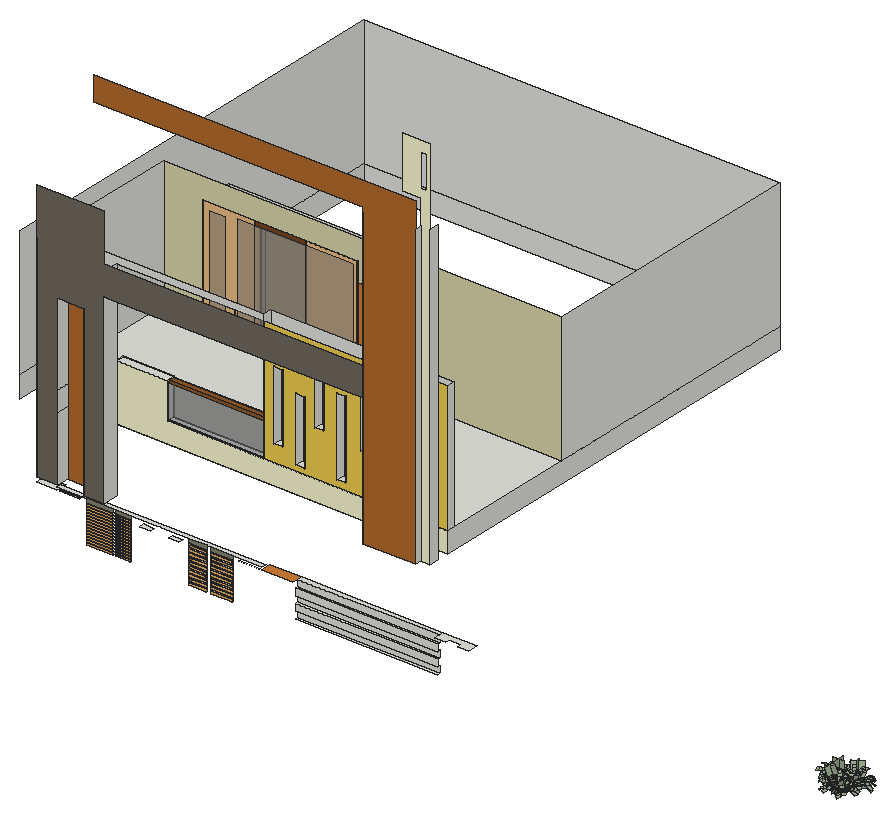
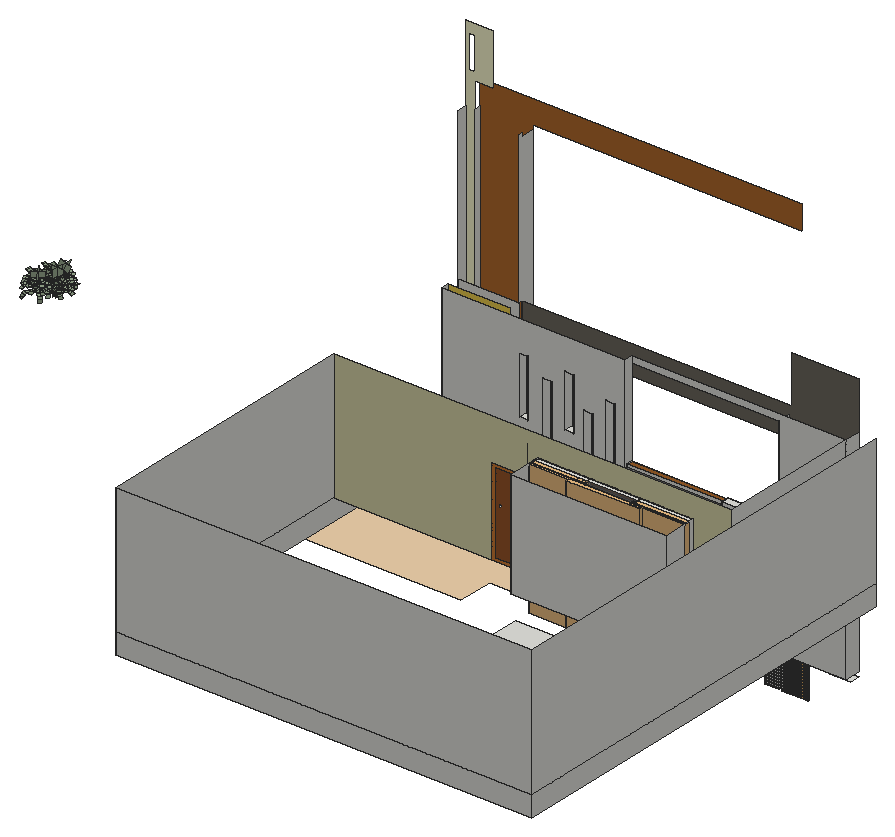
# SketchUp Ruby script. Lengths in inches.
U = 1.inch
M = Sketchup.active_model
def pt(a) = Geom::Point3d.new(a.map { |v| v * U })
def face(e, loops, mat)
  f = e.add_face(loops[0].map { |a| pt(a) })
  loops[1..].each { |l| e.add_face(l.map { |a| pt(a) }).erase! }
  f.material = f.back_material = mat if mat
  f
end
# faces: each face lists its corners as indices into pts; further lists are holes
def faces(e, pts, list, mat = nil) = list.each { |f| face(e, (f[0].is_a?(Array) ? f : [f]).map { |l| l.map { |i| pts[i] } }, mat) }
# xy, xz, yz: faces in a plane at the given z, y or x. An outline is a flat list of corners, or four numbers for a rectangle; further outlines are holes
def ring(l) = l.size == 4 ? [[l[0], l[1]], [l[2], l[1]], [l[2], l[3]], [l[0], l[3]]] : l.each_slice(2).to_a
def flat(e, list, mat, &to3) = list.each { |f| face(e, (f[0].is_a?(Array) ? f : [f]).map { |l| ring(l).map { |u, v| to3.(u, v) } }, mat) }
def xy(e, z, list, mat = nil) = flat(e, list, mat) { |x, y| [x, y, z] }
def xz(e, y, list, mat = nil) = flat(e, list, mat) { |x, z| [x, y, z] }
def yz(e, x, list, mat = nil) = flat(e, list, mat) { |y, z| [x, y, z] }
def lines(e, pts, list) = list.each { |a, b| e.add_line(pt(pts[a]), pt(pts[b])) }
# prism: a flat outline (further loops are holes) pulled along v
def prism(e, loops, v, mat = nil)
  f = face(e, loops, mat); d = Geom::Vector3d.new(v.map { |x| x * U })
  f.pushpull(f.normal.samedirection?(d) ? d.length : -d.length)
end
def box(e, o, s, mat = nil) = prism(e, [[o, [o[0] + s[0], o[1], o[2]], [o[0] + s[0], o[1] + s[1], o[2]], [o[0], o[1] + s[1], o[2]]]], [0, 0, s[2]], mat)
def at(x, y, z, deg = 0) = Geom::Transformation.translation(pt([x, y, z])) * Geom::Transformation.rotation(ORIGIN, Z_AXIS, deg.degrees)
def axes(o, x, y, z) = Geom::Transformation.new([*x, 0, *y, 0, *z, 0, *pt(o).to_a, 1])
def part(name) = M.definitions.add(name)
# library, detail: a bought-in or finely detailed component or shape, given as its bounding box
def library(name, o, s) = part(name).tap { |d| box(d.entities, o, s) }
def detail(e, o, s) = box(e.add_group.entities, o, s)
def put(e, d, t, mat = nil) = e.add_instance(d, t).tap { |i| i.material = mat if mat }
def group(e, t, mat = nil) = e.add_group.tap { |g| g.transformation = t; g.material = mat if mat }.entities
root = M.entities
M.materials.add("Generic").color = [133, 133, 113]
M.materials.add("Generic\#1").color = [235, 176, 99]
M.materials.add("Generic\#4").color = [217, 213, 170]
M.materials.add("Generic\#5").color = [237, 206, 80]
M.materials.add("Generic\#6").color = [239, 209, 171]
M.materials.add("Generic\#7").color = [249, 247, 208]
M.materials.add("[Brick Antique 01]").color = [179, 108, 46]
M.materials.add("[Cladding Weathered]").color = [111, 105, 96]
M.materials.add("[Translucent Glass Gray]").color = [128, 128, 128]
M.materials["[Translucent Glass Gray]"].alpha = 0.5
M.materials.add("[Wood Bamboo]").color = [206, 124, 53]
M.materials.add("[Wood Cherry Original]").color = [152, 86, 42]
M.materials.add("[Wood Floor Light]").color = [204, 176, 127]
M.materials.add("[Wood Floor Parquet]").color = [145, 89, 39]
M.materials.add("[Wood Veneer 01]").color = [119, 69, 36]
M.materials.add("hymenocallis littoralis").color = [156, 172, 146]
c1 = part("Group\#856")
xy(c1.entities,7.38,[[0,0,5.5,15.91]],"hymenocallis littoralis")
p = [[5.5,28.78,0],[5.5,26.79,3.44],[0,26.79,3.44],[0,28.78,0],[0,23.75,6],[5.5,23.75,6],
  [0,15.91,7.38],[5.5,15.91,7.38]]
faces(c1.entities,p,[[0,1,2,3],[4,2,1,5],[6,4,5,7]],"hymenocallis littoralis")
c2 = part("Group\#854")
xy(c2.entities,7.38,[[0,0,5.5,15.91],[0,15.91,5.5,23.87]],"hymenocallis littoralis")
p = [[5.5,31.07,4.3],[5.5,27.74,6.47],[0,27.74,6.47],[0,31.07,4.3],[0,23.87,7.38],[5.5,23.87,7.38]]
faces(c2.entities,p,[[0,1,2,3],[4,2,1,5]],"hymenocallis littoralis")
c3 = part("Group\#857")
xy(c3.entities,7.38,[[0,0,5.6,15.91]],"hymenocallis littoralis")
p = [[5.6,28.78,0],[5.6,26.79,3.44],[0,26.79,3.44],[0,28.78,0],[0,23.75,6],[5.6,23.75,6],
  [0,15.91,7.38],[5.6,15.91,7.38]]
faces(c3.entities,p,[[0,1,2,3],[4,2,1,5],[6,4,5,7]],"hymenocallis littoralis")
c4 = part("Group\#855")
put(c4.entities,c2,axes([6.09,8.57,-0.52],[0.446,0.85617,0.26089],[-0.18444,-0.19731,0.96283],[0.87582,-0.47754,0.0699]))
put(c4.entities,c2,axes([6.29,7.28,-1.71],[0.37058,0.92707,-0.05667],[-0.32382,0.19004,0.99128],[0.87712,-0.32925,0.34964]))
put(c4.entities,c2,axes([11.04,16.14,-0.7],[1,0,0],[0,0.16628,1.02662],[0,-1.18456,0.19186]))
c5 = part("Group\#860")
put(c5.entities,c1,axes([24.57,32.05,-1.76],[0.9552,-0.22102,-0.19681],[0.4036,0.95545,0.88585],[-0.00568,-0.67859,0.7345]))
put(c5.entities,c1,axes([23.95,29.24,-2.4],[0,1,0],[-0.76041,0,0.64945],[0.64945,0,0.76041]))
put(c5.entities,c1,axes([24.22,24.72,-0.48],[-0.70711,0.70711,0],[-0.32757,-0.32757,0.80237],[0.61237,0.61237,0.5]))
put(c5.entities,c2,axes([20.66,37.22,-0.63],[1.12361,0.03262,0.39091],[-0.43499,0.29739,0.78777],[0.09852,-1.27434,0.37535]))
put(c5.entities,c1,axes([28.75,24.45,-2.4],[-1,0,0],[0,-0.76041,0.64945],[0,0.64945,0.76041]))
put(c5.entities,c3,axes([30.4,30.98,-3.7],[0.65676,-0.72002,0.22414],[0.55667,0.66341,0.5],[-0.50871,-0.20361,0.83652]))
put(c5.entities,c3,axes([32.41,29.61,-3.7],[0.04029,-0.97372,0.22414],[0.85287,0.15038,0.5],[-0.52057,0.17102,0.83652]))
put(c5.entities,c1,axes([31.89,25.85,-1.76],[-0.92056,0.33739,-0.19681],[-0.5186,-0.89824,0.88585],[0.08952,0.67268,0.7345]))
put(c5.entities,c1,axes([25.55,34.78,-0.48],[0.86603,0.5,0],[-0.25,0.43301,0.86603],[0.43301,-0.75,0.5]))
put(c5.entities,c3,axes([20.4,16.9375,-8.07],[-0.70711,0.70711,0],[-0.35754,-0.35754,0.65422],[1.3987,1.3987,1.52882]))
put(c5.entities,c1,axes([32.86,34.14,-0.48],[0.76604,-0.64279,0],[0.32139,0.38302,0.86603],[-0.55667,-0.66341,0.5]))
put(c5.entities,c1,axes([27.15,34.7,-0.1],[0.82472,-0.17528,-0.53769],[0.53769,0.53769,0.64945],[0.17528,-0.82472,0.53769]))
put(c5.entities,c1,axes([33.58,28.77,-2.4],[0,-1,0],[0.76041,0,0.64945],[-0.64945,0,0.76041]))
put(c5.entities,c1,axes([26.43,23.87,-2.81],[-0.75126,0.04415,0.65853],[0.53769,-0.53769,0.64945],[0.38276,0.84199,0.3802]))
put(c5.entities,c1,axes([28.78,23.98,-2.4],[-1,0,0],[0,-0.76041,0.64945],[0,0.64945,0.76041]))
put(c5.entities,c1,axes([25.39,25.38,-2.4],[-0.70711,0.70711,0],[-0.53769,-0.53769,0.64945],[0.45923,0.45923,0.76041]))
put(c5.entities,c1,axes([27.32,21.63,-0.1],[-0.45923,0.70711,-0.53769],[-0.76041,0,0.64945],[0.45923,0.70711,0.53769]))
put(c5.entities,c1,axes([25.17,27.625,-1.76],[0.56416,0.80187,-0.19681],[-0.66673,0.66673,0.80532],[0.62659,-0.26057,0.7345]))
put(c5.entities,c3,axes([27.59,27.04,-3.96],[-0.8993,-0.06127,0.43301],[0.2962,-0.8138,0.5],[0.32175,0.57791,0.75]))
put(c5.entities,c3,axes([26.98,24.5,-3.18],[-0.5,0.86603,0],[-0.75,-0.43301,0.5],[0.43301,0.25,0.86603]))
put(c5.entities,c3,axes([24.55,27.74,-3.7],[0.29517,0.92878,0.22414],[-0.85287,0.15038,0.5],[0.43068,-0.33875,0.83652]))
put(c5.entities,c3,axes([24.26,29.8,-3.18],[0.76604,0.64279,0],[-0.47317,0.5639,0.425],[0.32139,-0.38302,0.86603]))
put(c5.entities,c3,axes([25.98,32.46,-3.18],[1,0,0],[0,0.86603,0.5],[0,-0.5,0.86603]))
put(c5.entities,c1,axes([28.78,33.57,-2.4],[1,0,0],[0,0.76041,0.64945],[0,-0.64945,0.76041]))
put(c5.entities,c4,at(14.99,21.38,2.5))
put(c5.entities,c2,axes([34.63,26.34,-1.46],[-0.70089,-0.70877,0.07994],[0.4756,-0.38088,0.79293],[-0.53156,0.59378,0.60405]))
put(c5.entities,c2,axes([28.14,16.92,1.8125],[-1.19719,0.6912,0],[-0.09607,-0.16641,0.94244],[0.68444,1.18549,0.17613]))
put(c5.entities,c2,axes([31.5625,35.84,0.97],[0.66765,-1.1564,0.35779],[0.04445,0.30732,0.91033],[-1.20828,-0.64496,0.17012]))
put(c5.entities,c2,axes([38.94,22.51,0.89],[-0.97932,-0.67164,-0.05202],[0.27787,-0.41401,0.90999],[-0.85985,0.93577,0.32097]))
put(c5.entities,c2,axes([38.44,21.09,1.98],[-1.02864,-0.54856,0.2395],[0.33481,0.06999,0.88388],[-0.77261,1.08328,0.06417]))
put(c5.entities,c3,axes([35.02,30.51,-1.3],[-0.17365,-0.98481,0],[0.60224,-0.10619,0.79122],[-0.7792,0.13739,0.61153]))
put(c5.entities,c3,axes([29.41,22.33,-1.3],[-0.93969,0.34202,0],[-0.20915,-0.57465,0.79122],[0.27061,0.74351,0.61153]))
put(c5.entities,c2,axes([19.64,36,-1.62],[1.18194,0.09546,0.08234],[-0.14377,0.68823,0.76313],[0.21457,-1.1326,0.62386]))
put(c5.entities,c3,axes([24.25,24.14,-1.3],[-0.34202,0.93969,0],[-0.57465,-0.20915,0.79122],[0.74351,0.27061,0.61153]))
put(c5.entities,c3,axes([25.98,34.61,-1.3],[1,0,0],[0,0.61153,0.79122],[0,-0.79122,0.61153]))
put(c5.entities,c3,axes([31.16,34.41,-1.64],[0.56518,-0.80224,-0.19234],[0.73413,0.34233,0.72935],[-0.47639,-0.50772,0.71782]))
put(c5.entities,c3,axes([40.52,26.84,-5.82],[-0.42262,-0.90631,0],[0.48019,-0.22391,0.68552],[-1.43418,0.66877,1.22305]))
put(c5.entities,c1,axes([29.86,38.42,-1.01],[0.89064,-0.37013,0.26413],[-0.03924,0.63286,1.01918],[-0.45353,-0.76487,0.45748]))
put(c5.entities,c1,axes([29.34,22.4,-0.48],[-0.99619,-0.08716,0],[0.04358,-0.4981,0.86603],[-0.07548,0.86273,0.5]))
c6 = part("Group\#858")
xz(c6.entities,10.07,[[9.07,0,10.07,31.01],[0,31.01,0,45.12,20.13,45.12,20.13,31.01,10.07,31.01,10.07,32.58,9.07,32.58,9.07,31.01]],"hymenocallis littoralis")
yz(c6.entities,10.07,[[0,31.01,20.13,45.12]],"hymenocallis littoralis")
p = [[9.57,9.2,0],[10.07,10.07,0],[10.07,10.07,31.01],[10.07,10.07,32.58],[9.57,9.2,32.58]]
faces(c6.entities,p,[[0,1,2,3,4]],"hymenocallis littoralis")
c7 = part("cây lá nắng")
put(c7.entities,c5,axes([49.26,-2.75,0],[0.63109,0.63109,0],[-0.63109,0.63109,0],[0,0,0.935]))
g1 = group(c7.entities,at(26.6,-8.68,0))
put(g1,c1,axes([-4.72,35.73,-1.65],[0.74231,0.46334,-0.18402],[-0.34827,0.85768,0.82827],[0.42467,-0.43184,0.68675]))
put(g1,c1,axes([-3.34,33.57,-2.24],[-0.63109,0.63109,0],[-0.47989,-0.47989,0.60723],[0.40986,0.40986,0.71098]))
put(g1,c1,axes([-0.3125,30.89,-0.45],[-0.8925,0,0],[0,-0.41345,0.75022],[0,0.77293,0.4675]))
put(g1,c2,axes([-10.79,39.66,-0.59],[0.68852,0.72969,0.3655],[-0.4622,-0.08684,0.73657],[0.86641,-0.74205,0.35095]))
put(g1,c1,axes([2.71,33.57,-2.24],[-0.63109,-0.63109,0],[0.47989,-0.47989,0.60723],[-0.40986,0.40986,0.71098]))
put(g1,c3,axes([-0.37,38.74,-3.46],[0.86887,-0.03992,0.20957],[-0.06737,0.76999,0.4675],[-0.19255,-0.44954,0.78214]))
put(g1,c3,axes([1.76,39.14,-3.46],[0.63993,-0.58908,0.20957],[0.44333,0.63315,0.4675],[-0.43646,-0.2206,0.78214]))
put(g1,c1,axes([3.81,36.4375,-1.65],[-0.79389,-0.36803,-0.18402],[0.23959,-0.89415,0.82827],[-0.36803,0.48102,0.68675]))
put(g1,c1,axes([-5.83,38.07,-0.45],[0.231,0.86209,0],[-0.43104,0.1155,0.80973],[0.74659,-0.20005,0.4675]))
put(g1,c3,axes([2.18,23.5625,-7.55],[-0.8925,0,0],[0,-0.45128,0.6117],[0,1.76542,1.42944]))
put(g1,c1,axes([-0.8125,42.28,-0.45],[0.8891,0.07779,0],[-0.03889,0.44455,0.80973],[0.06737,-0.76999,0.4675]))
put(g1,c1,axes([-4.76,39.03,-0.09],[0.63109,0.40986,-0.50274],[0,0.67866,0.60723],[0.63109,-0.40986,0.50274]))
put(g1,c1,axes([3.03,39.35,-2.24],[0.63109,-0.63109,0],[0.47989,0.47989,0.60723],[-0.40986,-0.40986,0.71098]))
put(g1,c1,axes([1.61,31.74,-2.625],[-0.50198,-0.44625,0.61573],[0.67866,0,0.60723],[-0.28982,0.77293,0.35549]))
put(g1,c1,axes([3.03,33.3,-2.24],[-0.63109,-0.63109,0],[0.47989,-0.47989,0.60723],[-0.40986,0.40986,0.71098]))
put(g1,c1,axes([0.01,32.04,-2.24],[-0.8925,0,0],[0,-0.67866,0.60723],[0,0.57963,0.71098]))
put(g1,c1,axes([3.59,30.89,-0.09],[-0.73607,0.15643,-0.50274],[-0.47989,-0.47989,0.60723],[-0.15643,0.73607,0.50274]))
put(g1,c1,axes([-1.55,33.32,-1.65],[-0.15002,0.86209,-0.18402],[-0.84154,0,0.75297],[0.55988,0.231,0.68675]))
put(g1,c3,axes([0.35,34.48,-3.71],[-0.52887,-0.60621,0.40487],[0.70051,-0.32665,0.4675],[-0.16166,0.56777,0.70125]))
put(g1,c3,axes([2.61,39.13,-1.74],[-0.86209,0.231,0],[-0.23031,-0.85954,0.15531],[0.03162,0.11799,0.91645]))
put(g1,c3,axes([-2.02,33,-3.46],[-0.39986,0.77243,0.20957],[-0.63315,-0.44333,0.4675],[0.48558,0.05802,0.78214]))
put(g1,c3,axes([-3.49,34.12,-2.97],[0.07779,0.8891,0],[-0.65449,0.05726,0.39737],[0.44455,-0.03889,0.80973]))
put(g1,c3,axes([-4.09,36.88,-2.97],[0.63109,0.63109,0],[-0.54654,0.54654,0.4675],[0.31555,-0.31555,0.80973]))
put(g1,c1,axes([-3.02,39.35,-2.24],[0.63109,0.63109,0],[-0.47989,0.47989,0.60723],[0.40986,-0.40986,0.71098]))
put(g1,c4,axes([-4.03,22.95,2.33],[0.63109,0.63109,0],[-0.63109,0.63109,0],[0,0,0.935]))
put(g1,c2,axes([5.24,38.48,-1.37],[0.00497,-0.88963,0.07474],[0.54052,0.05978,0.74139],[-0.71019,0.03927,0.56479]))
put(g1,c2,axes([7.08,28.4375,1.7],[-1.19175,-0.31933,0],[0.04439,-0.16565,0.88118],[-0.31621,1.1801,0.16468]))
put(g1,c2,axes([-2.7,42.54,0.91],[1.15114,-0.30845,0.33454],[-0.1659,0.22199,0.85115],[-0.3555,-1.16957,0.15907]))
put(g1,c2,axes([10.37,38.78,0.83],[-0.19417,-1.04191,-0.04864],[0.43664,-0.08592,0.85084],[-1.1332,0.04791,0.30011]))
put(g1,c2,axes([10.95,37.5625,1.85],[-0.30298,-0.99536,0.22393],[0.16713,0.25547,0.82643],[-1.17124,0.19607,0.06]))
put(g1,c3,axes([2.84,41.36,-1.22],[0.51192,-0.73109,0],[0.44708,0.31305,0.73979],[-0.57846,-0.40504,0.57178]))
put(g1,c3,axes([4.47,32.65,-1.22],[-0.80888,-0.37719,0],[0.23066,-0.49465,0.73979],[-0.29844,0.64,0.57178]))
put(g1,c2,axes([-10.32,35.12,-1.51],[0.68567,0.80616,0.07699],[-0.52507,0.3436,0.71352],[0.85019,-0.57936,0.58331]))
put(g1,c3,axes([0.07,30.54,-1.22],[-0.80888,0.37719,0],[-0.23066,-0.49465,0.73979],[0.29844,0.64,0.57178]))
put(g1,c3,axes([-5.45,38.24,-1.22],[0.63109,0.63109,0],[-0.38593,0.38593,0.73979],[0.49934,-0.49934,0.57178]))
put(g1,c3,axes([-2.05,41.38,-1.53],[0.86296,-0.14961,-0.17984],[0.24726,0.67935,0.68194],[0.01977,-0.62107,0.67116]))
put(g1,c3,axes([8.63,42.51,-5.4375],[0.30525,-0.83868,0],[0.44435,0.16173,0.64096],[-1.32716,-0.48305,1.14356]))
put(g1,c1,axes([-5.4,43.09,-0.94],[0.79566,0.32849,0.24696],[-0.42416,0.37462,0.95293],[0.19648,-0.76892,0.42774]))
put(g1,c1,axes([4.38,32.65,-0.45],[-0.57369,-0.68369,0],[0.34185,-0.28684,0.80973],[-0.5921,0.49683,0.4675]))
put(g1,c3,axes([-2,33.84,-0.15],[-0.24601,0.85793,0],[-0.85539,-0.24528,0.15531],[0.11742,0.03367,0.91645]))
put(g1,c3,axes([0.17,30.83,-4.47],[-0.24601,0.85793,0],[-0.85539,-0.24528,0.15531],[0.11742,0.03367,0.91645]))
put(g1,c3,axes([-1.97,32.18,-4.47],[0.58524,0.67383,0],[-0.67184,0.58351,0.15531],[0.09222,-0.0801,0.91645]))
put(g1,c3,axes([-2,34.71,-4.47],[0.88392,-0.12346,0],[0.12309,0.88131,0.15531],[-0.0169,-0.12098,0.91645]))
put(g1,c3,axes([0.11,36.12,-4.47],[0.37822,-0.8084,0],[0.80601,0.37711,0.15531],[-0.11064,-0.05177,0.91645]))
put(c7.entities,c6,axes([29.71,14.29,6.94],[0.425,0.73612,0],[-0.6771,0.39092,-0.33349],[-0.26859,0.15507,0.72712]))
put(c7.entities,c6,axes([42.0625,26.12,6.94],[0.85,0,0],[0,0.78185,-0.33349],[0,0.33349,0.78185]))
put(c7.entities,c5,axes([7.3125,23.0625,0],[0.8925,0,0],[0,0.8925,0],[0,0,0.935]))
put(c7.entities,c6,axes([24.4375,40.23,2.05],[0.85,0,0],[0,0.85,0],[0,0,0.85]))
c8 = part("Planting+101")
put(c8.entities,c7,axes([21.34,32.96,-4.59],[0,-0.71,0],[-0.71,0,0],[0,0,0.71]))
c9 = library("Group14",[-64.97,9.24,0.31],[138.52,9.93,292.57])
c10 = library("Group16",[86.37,-10.76,76.46],[21.79,14.87,35.97])
c11 = library("Group22",[48.82,-10.91,0.23],[97.72,18.57,293.12])
c12 = library("Group24",[44.03,2.01,0.26],[103.73,11,292.35])
c13 = library("Group27",[-106.21,-10.76,76.46],[21.8,14.87,35.97])
c14 = library("Group35",[-145.81,2.01,0.26],[103.73,11,292.35])
c15 = library("Group33",[-144.59,-10.91,0.23],[97.72,18.57,293.12])
c16 = part("rem (1)")
g2 = group(c16.entities,at(-145.81,-10.91,0.23))
put(g2,c9,at(145.81,10.91,-0.23))
put(g2,c10,at(145.81,10.91,-0.23))
put(g2,c11,at(145.81,10.91,-0.23))
put(g2,c12,at(145.81,10.91,-0.23))
put(g2,c13,at(145.81,10.91,-0.23))
put(g2,c14,at(145.81,10.91,-0.23))
put(g2,c15,at(145.81,10.91,-0.23))
xy(root,24.125,[[74.16,67.875,103.6875,68.625],[107.25,67.875,123.28,68.625]])
xy(root,24.1875,[[188.84,67.875,208,68.625],[212.8125,67.875,236.91,68.625]],"Generic")
xy(root,25.875,[[74.16,67.875,103.6875,68.625],[107.25,67.875,123.28,68.625]])
xy(root,26.5625,[[188.84,67.875,208,68.625],[212.8125,67.875,236.91,68.625]],"Generic")
xy(root,27.125,[[74.16,67.875,103.6875,68.625],[107.25,67.875,123.28,68.625]])
xy(root,28.375,[[188.84,67.875,208,68.625],[212.8125,67.875,236.91,68.625]],"Generic")
xy(root,28.875,[[74.16,67.875,103.6875,68.625],[107.25,67.875,123.28,68.625]])
xy(root,29.5625,[[304.6875,71.375,462.8125,74.375]])
xy(root,30.125,[[74.16,67.875,103.6875,68.625],[107.25,67.875,123.28,68.625]])
xy(root,30.75,[[188.84,67.875,208,68.625],[212.8125,67.875,236.91,68.625]],"Generic")
xy(root,31.875,[[74.16,67.875,103.6875,68.625],[107.25,67.875,123.28,68.625]])
xy(root,32.5625,[[188.84,67.875,208,68.625],[212.8125,67.875,236.91,68.625]],"Generic")
xy(root,33.125,[[74.16,67.875,103.6875,68.625],[107.25,67.875,123.28,68.625]])
xy(root,34.875,[[74.16,67.875,103.6875,68.625],[107.25,67.875,123.28,68.625]])
xy(root,34.9375,[[188.84,67.875,208,68.625],[212.8125,67.875,236.91,68.625]],"Generic")
xy(root,36.125,[[74.16,67.875,103.6875,68.625],[107.25,67.875,123.28,68.625]])
xy(root,36.75,[[188.84,67.875,208,68.625],[212.8125,67.875,236.91,68.625]],"Generic")
xy(root,37,[[304.6875,71.375,462.8125,74.375]])
xy(root,37.875,[[74.16,67.875,103.6875,68.625],[107.25,67.875,123.28,68.625]])
xy(root,39.125,[[74.16,67.875,103.6875,68.625],[107.25,67.875,123.28,68.625]])
xy(root,39.125,[[188.84,67.875,208,68.625],[212.8125,67.875,236.91,68.625]],"Generic")
xy(root,40.875,[[74.16,67.875,103.6875,68.625],[107.25,67.875,123.28,68.625]])
xy(root,40.9375,[[188.84,67.875,208,68.625],[212.8125,67.875,236.91,68.625]],"Generic")
xy(root,42.125,[[74.16,67.875,103.6875,68.625],[107.25,67.875,123.28,68.625]])
xy(root,43.3125,[[188.84,67.875,208,68.625],[212.8125,67.875,236.91,68.625]],"Generic")
xy(root,43.875,[[74.16,67.875,103.6875,68.625],[107.25,67.875,123.28,68.625]])
xy(root,44.875,[[304.6875,71.375,462.8125,74.375]])
xy(root,45.125,[[74.16,67.875,103.6875,68.625],[107.25,67.875,123.28,68.625]])
xy(root,45.125,[[188.84,67.875,208,68.625],[212.8125,67.875,236.91,68.625]],"Generic")
xy(root,46.875,[[74.16,67.875,103.6875,68.625],[107.25,67.875,123.28,68.625]])
xy(root,47.5,[[188.84,67.875,208,68.625],[212.8125,67.875,236.91,68.625]],"Generic")
xy(root,48.125,[[74.16,67.875,103.6875,68.625],[107.25,67.875,123.28,68.625]])
xy(root,49.3125,[[188.84,67.875,208,68.625],[212.8125,67.875,236.91,68.625]],"Generic")
xy(root,49.875,[[74.16,67.875,103.6875,68.625],[107.25,67.875,123.28,68.625]])
xy(root,51.125,[[74.16,67.875,103.6875,68.625],[107.25,67.875,123.28,68.625]])
xy(root,51.6875,[[188.84,67.875,208,68.625],[212.8125,67.875,236.91,68.625]],"Generic")
xy(root,52.3125,[[304.6875,71.375,462.8125,74.375]])
xy(root,52.875,[[74.16,67.875,103.6875,68.625],[107.25,67.875,123.28,68.625]])
xy(root,53.5,[[188.84,67.875,208,68.625],[212.8125,67.875,236.91,68.625]],"Generic")
xy(root,54.125,[[74.16,67.875,103.6875,68.625],[107.25,67.875,123.28,68.625]])
xy(root,55.875,[[74.16,67.875,103.6875,68.625],[107.25,67.875,123.28,68.625]])
xy(root,55.875,[[188.84,67.875,208,68.625],[212.8125,67.875,236.91,68.625]],"Generic")
xy(root,57.125,[[74.16,67.875,103.6875,68.625],[107.25,67.875,123.28,68.625]])
xy(root,57.6875,[[188.84,67.875,208,68.625],[212.8125,67.875,236.91,68.625]],"Generic")
xy(root,58.875,[[74.16,67.875,103.6875,68.625],[107.25,67.875,123.28,68.625]])
xy(root,60.0625,[[188.84,67.875,208,68.625],[212.8125,67.875,236.91,68.625]],"Generic")
xy(root,60.125,[[74.16,67.875,103.6875,68.625],[107.25,67.875,123.28,68.625]])
xy(root,60.1875,[[304.6875,71.375,462.8125,74.375]])
xy(root,61.875,[[74.16,67.875,103.6875,68.625],[107.25,67.875,123.28,68.625]])
xy(root,61.875,[[188.84,67.875,208,68.625],[212.8125,67.875,236.91,68.625]],"Generic")
xy(root,62.9375,[[166.3125,67.875,177.72,72.625]])
xy(root,63.125,[[74.16,67.875,103.6875,68.625],[107.25,67.875,123.28,68.625]])
xy(root,63.46,[[134.26,67.875,145.71,72.625]])
xy(root,64.25,[[188.84,67.875,208,68.625],[212.8125,67.875,236.91,68.625]],"Generic")
xy(root,64.875,[[74.16,67.875,103.6875,68.625],[107.25,67.875,123.28,68.625]])
xy(root,66.0625,[[188.84,67.875,208,68.625],[212.8125,67.875,236.91,68.625]])
xy(root,66.125,[[74.16,67.875,103.6875,68.625],[107.25,67.875,123.28,68.625]])
xy(root,67.5,[[19.1875,67.875,41.625,79.3125],[462.8125,67.875,475.25,67.875,475.25,73.0625,487.6875,73.0625,487.6875,67.875,500.125,67.875,500.125,79.3125,462.8125,79.3125],[304.6875,74.375,462.8125,79.3125]])
xy(root,67.5,[[269.875,67.875,304.6875,79.3125]],"[Wood Bamboo]")
xy(root,67.73,[[244.11,67.875,267.11,68.625]])
xy(root,67.76,[[44.36,67.875,67.42,68.625]])
xy(root,70.5,[[41.625,67.875,152.75,67.875,152.75,68.625,158.75,68.625,158.75,67.875,269.875,67.875,269.875,72.625,41.625,72.625]])
xy(root,72.125,[[19.1875,67.875,19.1875,85.3125,93.91,85.3125,93.91,67.875,71.06,67.875,71.06,81.625,42.04,81.625,42.04,67.875]])
xy(root,115.9375,[[43.125,244.125,260.5625,338.6875]])
xy(root,144,[[394.04,53.25,394.04,72.375,462.8125,72.375,462.8125,60.6875,452.8125,60.6875,452.8125,53.25]])
xy(root,144,[[19.1875,85.3125,19.1875,244.125,288.89,244.125,288.89,284.5625,462.8125,284.5625,462.8125,85.3125]],"Generic\#6")
xy(root,167.1875,[[19.1875,85.3125,19.1875,244.125,62.44,244.125,62.44,281.25,235.88,281.25,235.88,244.125,462.8125,244.125,462.8125,94.5625,93.91,94.5625,93.91,85.3125],[150.8,85.3125,150.8,86.72,256.84,86.72,256.84,93.15,150.8,93.15,150.8,94.5625,258.25,94.5625,258.25,85.3125],[258.25,85.3125,462.8125,94.5625],[150.8,86.72,256.84,93.15]])
xy(root,173.22,[[294.23,85.3125,304.04,94.5625]])
xy(root,174.68,[[339.93,85.3125,349.75,94.5625]])
xy(root,185.81,[[269.72,85.3125,279.54,94.5625]])
xy(root,204.125,[[150.8,86.72,256.84,93.15]])
xy(root,207.4375,[[93.91,85.3125,150.8,94.5625]])
xy(root,207.4375,[[150.8,86.72,256.84,93.15]],"[Wood Floor Parquet]")
xy(root,212.98,[[366.08,85.3125,375.89,94.5625]])
xy(root,217.99,[[315.33,85.3125,325.14,94.5625]])
xz(root,53.25,[[394.04,144,452.8125,144,452.8125,506.6875,93.91,506.6875,93.91,480.125,394.04,480.125]],"[Brick Antique 01]")
xz(root,60.6875,[[[452.8125,144,462.8125,144,462.8125,564.0625,432.56,564.0625,432.56,506.6875,452.8125,506.6875],[452.8125,515.875,459.25,552.5]]],"Generic\#7")
xz(root,67.875,[[188.84,66.0625,208,70.5],[212.8125,66.0625,236.91,70.5],[74.16,66.125,103.6875,70.5],[107.25,66.125,123.28,70.5]],"Generic")
xz(root,67.875,[[74.16,24.125,103.6875,25.875],[107.25,24.125,123.28,25.875],[188.84,24.1875,208,26.5625],[212.8125,24.1875,236.91,26.5625],[74.16,27.125,103.6875,28.875],
  [107.25,27.125,123.28,28.875],[188.84,28.375,208,30.75],[212.8125,28.375,236.91,30.75],[74.16,30.125,103.6875,31.875],[107.25,30.125,123.28,31.875],
  [188.84,32.5625,208,34.9375],[212.8125,32.5625,236.91,34.9375],[74.16,33.125,103.6875,34.875],[107.25,33.125,123.28,34.875],[74.16,36.125,103.6875,37.875],
  [107.25,36.125,123.28,37.875],[188.84,36.75,208,39.125],[212.8125,36.75,236.91,39.125],[74.16,39.125,103.6875,40.875],[107.25,39.125,123.28,40.875],
  [188.84,40.9375,208,43.3125],[212.8125,40.9375,236.91,43.3125],[74.16,42.125,103.6875,43.875],[107.25,42.125,123.28,43.875],[74.16,45.125,103.6875,46.875],
  [107.25,45.125,123.28,46.875],[188.84,45.125,208,47.5],[212.8125,45.125,236.91,47.5],[74.16,48.125,103.6875,49.875],[107.25,48.125,123.28,49.875],
  [188.84,49.3125,208,51.6875],[212.8125,49.3125,236.91,51.6875],[74.16,51.125,103.6875,52.875],[107.25,51.125,123.28,52.875],[188.84,53.5,208,55.875],
  [212.8125,53.5,236.91,55.875],[74.16,54.125,103.6875,55.875],[107.25,54.125,123.28,55.875],[74.16,57.125,103.6875,58.875],[107.25,57.125,123.28,58.875],
  [188.84,57.6875,208,60.0625],[212.8125,57.6875,236.91,60.0625],[74.16,60.125,103.6875,61.875],[107.25,60.125,123.28,61.875],[188.84,61.875,208,64.25],
  [212.8125,61.875,236.91,64.25],[74.16,63.125,103.6875,64.875],[107.25,63.125,123.28,64.875]],"Generic\#1")
xz(root,67.875,[[19.1875,72.125,42.04,72.125,42.04,258.96,71.06,258.96,71.06,72.125,93.91,72.125,93.91,278.625,394.04,278.625,394.04,311.1875,93.91,311.1875,93.91,364.3125,19.1875,364.3125]],"[Cladding Weathered]")
xz(root,68.625,[[74.16,25.875,103.6875,27.125],[107.25,25.875,123.28,27.125],[188.84,26.5625,208,28.375],[212.8125,26.5625,236.91,28.375],[74.16,28.875,103.6875,30.125],
  [107.25,28.875,123.28,30.125],[188.84,30.75,208,32.5625],[212.8125,30.75,236.91,32.5625],[74.16,31.875,103.6875,33.125],[107.25,31.875,123.28,33.125],
  [74.16,34.875,103.6875,36.125],[107.25,34.875,123.28,36.125],[188.84,34.9375,208,36.75],[212.8125,34.9375,236.91,36.75],[74.16,37.875,103.6875,39.125],
  [107.25,37.875,123.28,39.125],[188.84,39.125,208,40.9375],[212.8125,39.125,236.91,40.9375],[74.16,40.875,103.6875,42.125],[107.25,40.875,123.28,42.125],
  [188.84,43.3125,208,45.125],[212.8125,43.3125,236.91,45.125],[74.16,43.875,103.6875,45.125],[107.25,43.875,123.28,45.125],[74.16,46.875,103.6875,48.125],
  [107.25,46.875,123.28,48.125],[188.84,47.5,208,49.3125],[212.8125,47.5,236.91,49.3125],[74.16,49.875,103.6875,51.125],[107.25,49.875,123.28,51.125],
  [188.84,51.6875,208,53.5],[212.8125,51.6875,236.91,53.5],[74.16,52.875,103.6875,54.125],[107.25,52.875,123.28,54.125],[74.16,55.875,103.6875,57.125],
  [107.25,55.875,123.28,57.125],[188.84,55.875,208,57.6875],[212.8125,55.875,236.91,57.6875],[74.16,58.875,103.6875,60.125],[107.25,58.875,123.28,60.125],
  [188.84,60.0625,208,61.875],[212.8125,60.0625,236.91,61.875],[74.16,61.875,103.6875,63.125],[107.25,61.875,123.28,63.125],[188.84,64.25,208,66.0625],
  [212.8125,64.25,236.91,66.0625],[74.16,64.875,103.6875,66.125],[107.25,64.875,123.28,66.125]])
xz(root,71.375,[[304.6875,37,462.8125,44.875],[304.6875,52.3125,462.8125,60.1875]])
xz(root,72.375,[[394.04,144,462.8125,311.1875]])
xz(root,74.375,[[304.6875,29.5625,462.8125,37],[304.6875,44.875,462.8125,52.3125],[304.6875,60.1875,462.8125,67.5]])
xz(root,81.625,[[42.04,72.125,71.06,258.96]],"[Brick Antique 01]")
xz(root,85.3125,[[19.1875,72.125,93.91,144],[19.1875,144,93.91,167.1875],[19.1875,167.1875,19.1875,311.1875,258.25,311.1875,258.25,304.1875,93.91,304.1875,93.91,167.1875]])
xz(root,85.3125,[[[258.25,167.1875,462.8125,167.1875,462.8125,311.1875,394.04,311.1875,394.04,304.1875,258.25,304.1875],[339.93,174.68,349.75,261.43],[269.72,185.81,279.54,263.68],[294.23,173.22,304.04,245.22],[366.08,212.98,375.89,277.23],[315.33,217.99,325.14,276.62]]],"Generic\#5")
xz(root,85.3125,[[93.91,144,462.8125,144,462.8125,167.1875,150.8,167.1875,150.8,207.4375,93.91,207.4375]],"Generic\#7")
xz(root,86.72,[[150.8,167.1875,256.84,204.125]],"[Translucent Glass Gray]")
xz(root,86.72,[[150.8,204.125,256.84,207.4375]],"[Wood Floor Parquet]")
xz(root,93.15,[[150.8,204.125,256.84,207.4375]])
xz(root,93.15,[[150.8,167.1875,256.84,204.125]],"[Translucent Glass Gray]")
xz(root,94.5625,[[93.91,167.1875,150.8,207.4375],[[258.25,167.1875,462.8125,311.1875],[339.93,174.68,349.75,261.43],[269.72,185.81,279.54,263.68],[294.23,173.22,304.04,245.22],[366.08,212.98,375.89,277.23],[315.33,217.99,325.14,276.62]]])
xz(root,244.125,[[19.1875,167.1875,62.44,167.1875,62.44,286.8125,235.88,286.8125,235.88,264.58,286.57,264.58,286.57,167.1875,462.8125,167.1875,462.8125,311.1875,19.1875,311.1875]],"Generic\#4")
xz(root,244.125,[[[235.88,167.1875,286.57,264.58],[240.0625,171.37,282.39,260.39]]],"[Wood Bamboo]")
xz(root,244.125,[[[240.0625,171.37,282.39,260.39],[244.91,178.22,251.79,251.91],[277.8,222.23,277.28,222.3,276.8,222.5,276.38,222.8125,276.07,223.23,275.87,223.71,275.8,224.23,275.87,224.74,276.07,225.23,276.38,225.64,276.8,225.96,277.28,226.16,277.8,226.23,278.32,226.16,278.8,225.96,279.21,225.64,279.53,225.23,279.73,224.74,279.8,224.23,279.73,223.71,279.53,223.23,279.21,222.8125,278.8,222.5,278.32,222.3]]],"[Wood Cherry Original]")
xz(root,244.125,[[244.91,178.22,251.79,251.91]],"[Wood Floor Light]")
xz(root,281.25,[[62.44,167.1875,235.88,286.8125]])
xz(root,547.875,[[0,144,462.8125,167.1875],[0,167.1875,462.8125,311.1875]])
yz(root,0,[[67.875,144,547.875,167.1875],[67.875,167.1875,547.875,311.1875]])
yz(root,19.1875,[[67.875,72.125,85.3125,144],[67.875,144,85.3125,167.1875],[67.875,167.1875,85.3125,311.1875],[85.3125,167.1875,244.125,311.1875]])
yz(root,42.04,[[67.875,72.125,81.625,144],[67.875,144,81.625,167.1875],[67.875,167.1875,81.625,258.96]])
yz(root,62.44,[[244.125,167.1875,281.25,286.8125]])
yz(root,71.06,[[67.875,72.125,81.625,258.96]])
yz(root,74.16,[[67.875,25.875,68.625,27.125],[67.875,28.875,68.625,30.125],[67.875,31.875,68.625,33.125],[67.875,34.875,68.625,36.125],[67.875,37.875,68.625,39.125],
  [67.875,40.875,68.625,42.125],[67.875,43.875,68.625,45.125],[67.875,46.875,68.625,48.125],[67.875,49.875,68.625,51.125],[67.875,52.875,68.625,54.125],
  [67.875,55.875,68.625,57.125],[67.875,58.875,68.625,60.125],[67.875,61.875,68.625,63.125],[67.875,64.875,68.625,66.125]])
yz(root,93.91,[[67.875,72.125,85.3125,72.125,85.3125,304.1875,72.375,304.1875,72.375,278.625,67.875,278.625],[85.3125,167.1875,94.5625,207.4375]])
yz(root,103.6875,[[67.875,25.875,68.625,27.125],[67.875,28.875,68.625,30.125],[67.875,31.875,68.625,33.125],[67.875,34.875,68.625,36.125],[67.875,37.875,68.625,39.125],
  [67.875,40.875,68.625,42.125],[67.875,43.875,68.625,45.125],[67.875,46.875,68.625,48.125],[67.875,49.875,68.625,51.125],[67.875,52.875,68.625,54.125],
  [67.875,55.875,68.625,57.125],[67.875,58.875,68.625,60.125],[67.875,61.875,68.625,63.125],[67.875,64.875,68.625,66.125]])
yz(root,107.25,[[67.875,25.875,68.625,27.125],[67.875,28.875,68.625,30.125],[67.875,31.875,68.625,33.125],[67.875,34.875,68.625,36.125],[67.875,37.875,68.625,39.125],
  [67.875,40.875,68.625,42.125],[67.875,43.875,68.625,45.125],[67.875,46.875,68.625,48.125],[67.875,49.875,68.625,51.125],[67.875,52.875,68.625,54.125],
  [67.875,55.875,68.625,57.125],[67.875,58.875,68.625,60.125],[67.875,61.875,68.625,63.125],[67.875,64.875,68.625,66.125]])
yz(root,123.28,[[67.875,25.875,68.625,27.125],[67.875,28.875,68.625,30.125],[67.875,31.875,68.625,33.125],[67.875,34.875,68.625,36.125],[67.875,37.875,68.625,39.125],
  [67.875,40.875,68.625,42.125],[67.875,43.875,68.625,45.125],[67.875,46.875,68.625,48.125],[67.875,49.875,68.625,51.125],[67.875,52.875,68.625,54.125],
  [67.875,55.875,68.625,57.125],[67.875,58.875,68.625,60.125],[67.875,61.875,68.625,63.125],[67.875,64.875,68.625,66.125]])
yz(root,150.8,[[85.3125,167.1875,86.72,207.4375],[86.72,167.1875,93.15,204.125],[93.15,167.1875,94.5625,207.4375],[86.72,204.125,93.15,207.4375]])
yz(root,188.84,[[67.875,26.5625,68.625,28.375],[67.875,30.75,68.625,32.5625],[67.875,34.9375,68.625,36.75],[67.875,39.125,68.625,40.9375],[67.875,43.3125,68.625,45.125],
  [67.875,47.5,68.625,49.3125],[67.875,51.6875,68.625,53.5],[67.875,55.875,68.625,57.6875],[67.875,60.0625,68.625,61.875],[67.875,64.25,68.625,66.0625]])
yz(root,208,[[67.875,26.5625,68.625,28.375],[67.875,30.75,68.625,32.5625],[67.875,34.9375,68.625,36.75],[67.875,39.125,68.625,40.9375],[67.875,43.3125,68.625,45.125],
  [67.875,47.5,68.625,49.3125],[67.875,51.6875,68.625,53.5],[67.875,55.875,68.625,57.6875],[67.875,60.0625,68.625,61.875],[67.875,64.25,68.625,66.0625]])
yz(root,212.8125,[[67.875,26.5625,68.625,28.375],[67.875,30.75,68.625,32.5625],[67.875,34.9375,68.625,36.75],[67.875,39.125,68.625,40.9375],[67.875,43.3125,68.625,45.125],
  [67.875,47.5,68.625,49.3125],[67.875,51.6875,68.625,53.5],[67.875,55.875,68.625,57.6875],[67.875,60.0625,68.625,61.875],[67.875,64.25,68.625,66.0625]])
yz(root,235.88,[[244.125,167.1875,281.25,286.8125]])
yz(root,236.91,[[67.875,26.5625,68.625,28.375],[67.875,30.75,68.625,32.5625],[67.875,34.9375,68.625,36.75],[67.875,39.125,68.625,40.9375],[67.875,43.3125,68.625,45.125],
  [67.875,47.5,68.625,49.3125],[67.875,51.6875,68.625,53.5],[67.875,55.875,68.625,57.6875],[67.875,60.0625,68.625,61.875],[67.875,64.25,68.625,66.0625]])
yz(root,256.84,[[86.72,167.1875,93.15,204.125],[86.72,204.125,93.15,207.4375]])
yz(root,258.25,[[85.3125,167.1875,94.5625,311.1875]])
yz(root,269.72,[[85.3125,185.81,94.5625,263.68]])
yz(root,279.54,[[85.3125,185.81,94.5625,263.68]])
yz(root,294.23,[[85.3125,173.22,94.5625,245.22]])
yz(root,304.04,[[85.3125,173.22,94.5625,245.22]])
yz(root,315.33,[[85.3125,217.99,94.5625,276.62]])
yz(root,325.14,[[85.3125,217.99,94.5625,276.62]])
yz(root,339.93,[[85.3125,174.68,94.5625,261.43]])
yz(root,349.75,[[85.3125,174.68,94.5625,261.43]])
yz(root,366.08,[[85.3125,212.98,94.5625,277.23]])
yz(root,375.89,[[85.3125,212.98,94.5625,277.23]])
yz(root,394.04,[[53.25,144,53.25,474.875,67.875,474.875,67.875,478.375,72.375,478.375,72.375,311.1875,67.875,311.1875,67.875,278.625,72.375,278.625,72.375,144]])
yz(root,452.8125,[[53.25,144,60.6875,478.375]])
yz(root,462.8125,[[60.6875,144,72.375,478.375],[85.3125,144,547.875,167.1875],[85.3125,167.1875,94.5625,311.1875],[244.125,167.1875,547.875,311.1875]])
p = [[238.01,255.51,185.77],[238.01,255.51,305.4]]
lines(root,p,[[0,1]])
put(root,c8,at(957.82,18.4375,109.49))
put(root,c16,axes([148.58,249.6875,137.2],[0.59078,0,0],[0,0.51,0],[0,0,0.51]))
g3 = group(root,at(62.44,244.125,167.1875))
xy(g3,0,[[0,0,173.4375,5]])
xy(g3,119.625,[[0,0,173.4375,5]])
xz(g3,0,[[39.54,5.11,168.33,114.52],[7.87,7.87,26.57,111.75]],"[Translucent Glass Gray]")
xz(g3,0,[[[0,0,34.4375,119.625],[7.87,7.87,26.57,111.75]],[[34.4375,0,173.4375,119.625],[39.54,5.11,168.33,114.52]]],"[Wood Veneer 01]")
xz(g3,5,[[0,0,173.4375,119.625]],"[Translucent Glass Gray]")
yz(g3,0,[[0,0,5,119.625]])
yz(g3,173.4375,[[0,0,5,97.39],[0,97.39,5,119.625]])
